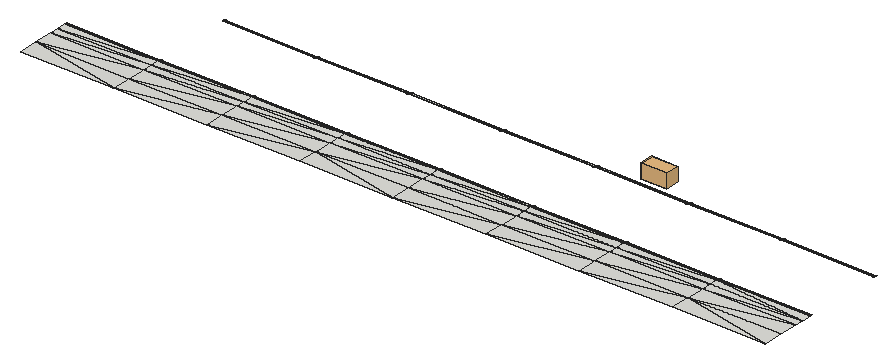
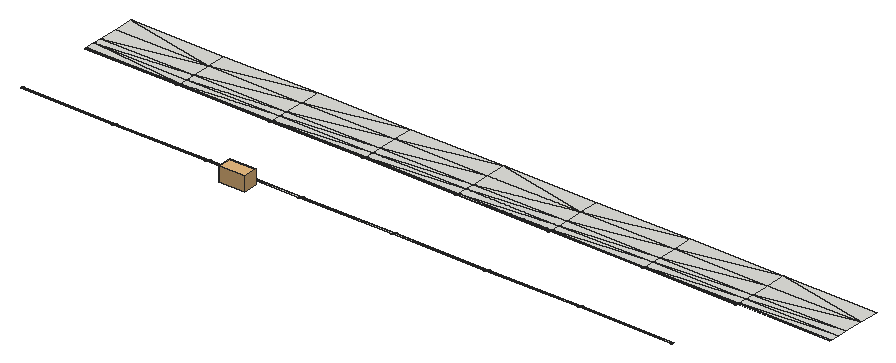
# SketchUp Ruby script. Lengths in inches.
U = 1.inch
M = Sketchup.active_model
def pt(a) = Geom::Point3d.new(a.map { |v| v * U })
def face(e, loops, mat)
  f = e.add_face(loops[0].map { |a| pt(a) })
  loops[1..].each { |l| e.add_face(l.map { |a| pt(a) }).erase! }
  f.material = f.back_material = mat if mat
  f
end
# faces: each face lists its corners as indices into pts; further lists are holes
def faces(e, pts, list, mat = nil) = list.each { |f| face(e, (f[0].is_a?(Array) ? f : [f]).map { |l| l.map { |i| pts[i] } }, mat) }
# xy, xz, yz: faces in a plane at the given z, y or x. An outline is a flat list of corners, or four numbers for a rectangle; further outlines are holes
def ring(l) = l.size == 4 ? [[l[0], l[1]], [l[2], l[1]], [l[2], l[3]], [l[0], l[3]]] : l.each_slice(2).to_a
def flat(e, list, mat, &to3) = list.each { |f| face(e, (f[0].is_a?(Array) ? f : [f]).map { |l| ring(l).map { |u, v| to3.(u, v) } }, mat) }
def xy(e, z, list, mat = nil) = flat(e, list, mat) { |x, y| [x, y, z] }
def xz(e, y, list, mat = nil) = flat(e, list, mat) { |x, z| [x, y, z] }
def yz(e, x, list, mat = nil) = flat(e, list, mat) { |y, z| [x, y, z] }
def lines(e, pts, list) = list.each { |a, b| e.add_line(pt(pts[a]), pt(pts[b])) }
# prism: a flat outline (further loops are holes) pulled along v
def prism(e, loops, v, mat = nil)
  f = face(e, loops, mat); d = Geom::Vector3d.new(v.map { |x| x * U })
  f.pushpull(f.normal.samedirection?(d) ? d.length : -d.length)
end
def box(e, o, s, mat = nil) = prism(e, [[o, [o[0] + s[0], o[1], o[2]], [o[0] + s[0], o[1] + s[1], o[2]], [o[0], o[1] + s[1], o[2]]]], [0, 0, s[2]], mat)
def at(x, y, z, deg = 0) = Geom::Transformation.translation(pt([x, y, z])) * Geom::Transformation.rotation(ORIGIN, Z_AXIS, deg.degrees)
def axes(o, x, y, z) = Geom::Transformation.new([*x, 0, *y, 0, *z, 0, *pt(o).to_a, 1])
def part(name) = M.definitions.add(name)
# library, detail: a bought-in or finely detailed component or shape, given as its bounding box
def library(name, o, s) = part(name).tap { |d| box(d.entities, o, s) }
def detail(e, o, s) = box(e.add_group.entities, o, s)
def put(e, d, t, mat = nil) = e.add_instance(d, t).tap { |i| i.material = mat if mat }
def group(e, t, mat = nil) = e.add_group.tap { |g| g.transformation = t; g.material = mat if mat }.entities
root = M.entities
c1 = library("Ruscus aculeatus 004",[-18.74,-17.86,-1.06],[37.01,36.62,28.95])
xy(root,0.2,[[0,116.21,0.61,116.21,0,116.39],[0.61,116.21,0.61,116.39,0,116.39]])
xy(root,0.37,[[1538.23,281.6,1539,281.6,1538.23,281.84],[1539,281.6,1539,281.84,1538.23,281.84],[1538.23,281.84,1539,281.84,1538.23,285.35],[1539,281.84,1539,285.35,1538.23,285.35],[1538.23,285.35,1539,285.35,1538.23,285.61],
  [1539,285.35,1539,285.61,1538.23,285.61]])
xy(root,0.375,[[1538.36,116.21,1539,116.21,1538.36,116.39],[1539,116.21,1539,116.39,1538.36,116.39],[1538.36,116.39,1539,116.39,1538.36,119.84],[1539,116.39,1539,119.84,1538.36,119.84],[1538.36,119.84,1539,119.84,1538.36,120.23],
  [1539,119.84,1539,120.23,1538.36,120.23]])
p = [[192.375,0,0.22],[192.375,40.18,0.22],[0,40.18,0.2],[0,0,0.2],[384.75,40.18,0.24],[384.75,0,0.24],
  [577.125,40.18,0.26],[577.125,0,0.27],[192.375,78.07,0.22],[0,78.07,0.2],[384.75,78.07,0.24],[577.125,78.07,0.26],
  [192.375,96.84,0.22],[0,96.84,0.2],[384.75,96.84,0.24],[577.125,96.84,0.26],[192.375,115.6,0.22],[0,115.6,0.2],
  [384.75,115.6,0.24],[577.125,115.6,0.26],[0,115.83,0.2],[192.375,115.83,0.22],[384.75,115.83,0.24],[577.125,115.83,0.26],
  [1154.25,115.83,0.33],[1154.25,115.97,0.22],[961.88,115.97,0.2],[961.88,115.83,0.31],[1346.63,115.83,0.35],[1346.63,115.97,0.24],
  [1539,115.83,0.375],[1539,115.97,0.27],[961.875,116.08,0.2],[961.875,116.21,0.31],[769.5,116.21,0.29],[1154.25,116.08,0.22],
  [1154.25,116.21,0.33],[1346.625,116.08,0.24],[1346.625,116.21,0.35],[1538.36,116.08,0.27],[1538.36,116.21,0.375],[192.375,116.21,0.22],
  [192.375,116.39,0.22],[0.61,116.39,0.2],[0.61,116.21,0.2],[384.75,116.39,0.24],[384.75,116.21,0.24],[577.125,116.39,0.26],
  [577.125,116.21,0.26],[0.61,119.84,0.19],[384.75,119.84,0.24],[192.375,119.84,0.22],[577.125,119.84,0.26],[192.375,120.23,0.22],
  [384.75,120.23,0.24],[577.125,120.23,0.26],[577.125,120.47,0.21],[769.5,120.23,0.28],[769.5,120.47,0.23],[961.875,120.23,0.31],
  [961.875,120.47,0.26],[577.125,281.36,0.21],[577.125,281.6,0.26],[384.75,281.6,0.24],[769.5,281.36,0.23],[769.5,281.6,0.28],
  [961.875,281.36,0.25],[384.75,281.84,0.24],[192.375,281.84,0.21],[192.375,281.6,0.21],[577.125,281.84,0.26],[384.75,285.35,0.24],
  [192.375,285.35,0.21],[577.125,285.35,0.26],[192.375,285.61,0.21],[384.75,285.61,0.24],[577.125,285.61,0.26],[1346.625,285.61,0.35],
  [1346.625,285.75,0.24],[1154.25,285.75,0.22],[1154.25,285.61,0.33],[1538.23,285.61,0.37],[1538.23,285.75,0.26],[769.5,0,0.29],
  [769.5,40.18,0.29],[961.875,40.18,0.31],[961.88,0,0.3125],[1154.25,40.18,0.33],[1154.25,0,0.33],[1346.63,40.18,0.35],
  [1346.63,0,0.36],[769.5,78.07,0.29],[961.875,78.07,0.31],[1154.25,78.07,0.33],[1346.63,78.07,0.35],[769.5,96.84,0.29],
  [961.875,96.84,0.31],[1154.25,96.84,0.33],[1346.63,96.84,0.35],[769.5,115.6,0.29],[961.88,115.6,0.31],[1154.25,115.6,0.33],
  [1346.63,115.6,0.35],[769.5,115.83,0.29],[1539,116.08,0.27],[1539,116.21,0.375],[769.5,116.39,0.29],[961.875,116.39,0.31],
  [1154.25,116.39,0.33],[1346.625,116.39,0.35],[769.5,119.84,0.28],[961.875,119.84,0.31],[1154.25,119.84,0.33],[1346.625,119.84,0.35],
  [1154.25,120.23,0.33],[1346.625,120.23,0.35],[1154.25,120.47,0.28],[1346.625,120.47,0.3],[1538.36,120.23,0.375],[1538.36,120.47,0.32],
  [1539,120.23,0.375],[1539,120.47,0.32],[961.875,281.6,0.3],[1154.25,281.36,0.28],[1154.25,281.6,0.33],[1346.63,281.36,0.3],
  [1346.63,281.6,0.35],[1538.23,281.36,0.32],[1538.23,281.6,0.37],[1539,281.36,0.32],[1539,281.6,0.37],[769.5,281.84,0.28],
  [961.875,281.84,0.3],[1154.25,281.84,0.33],[1346.63,281.84,0.35],[1538.23,281.84,0.37],[769.5,285.35,0.28],[961.875,285.35,0.3],
  [1154.25,285.35,0.33],[1346.625,285.35,0.35],[1538.23,285.35,0.37],[769.5,285.61,0.28],[961.875,285.61,0.3],[1539,285.61,0.37],
  [1539,285.75,0.26],[1539,0,0.38],[1539,40.18,0.38],[1539,78.07,0.375],[1539,96.84,0.375],[1539,115.6,0.375],
  [1538.36,116.39,0.375],[1538.36,119.84,0.375]]
faces(root,p,[[0,1,2],[2,3,0],[4,1,0],[0,5,4],[6,4,5],[5,7,6],[8,9,2],[2,1,8],
  [10,8,1],[1,4,10],[11,10,4],[4,6,11],[12,13,9],[9,8,12],[14,12,8],[8,10,14],
  [15,14,10],[10,11,15],[16,17,13],[13,12,16],[18,16,12],[12,14,18],[19,18,14],[14,15,19],
  [20,17,16],[16,21,20],[21,16,18],[18,22,21],[22,18,19],[19,23,22],[24,25,26],[26,27,24],
  [28,29,25],[25,24,28],[30,31,29],[29,28,30],[32,33,34],[33,32,35],[35,36,33],[36,35,37],
  [37,38,36],[37,39,40],[40,38,37],[41,42,43],[43,44,41],[45,42,41],[41,46,45],[47,45,46],
  [46,48,47],[49,43,42],[50,51,42],[42,45,50],[52,50,45],[45,47,52],[53,51,50],[50,54,53],
  [54,50,52],[52,55,54],[56,55,57],[57,58,56],[58,57,59],[59,60,58],[61,62,63],[62,61,64],
  [64,65,62],[65,64,66],[67,68,69],[69,63,67],[70,67,63],[63,62,70],[71,72,68],[68,67,71],
  [73,71,67],[67,70,73],[74,72,71],[71,75,74],[75,71,73],[73,76,75],[77,78,79],[79,80,77],
  [78,77,81],[81,82,78],[83,84,6],[6,7,83],[85,84,83],[83,86,85],[87,85,86],[86,88,87],
  [89,87,88],[88,90,89],[91,11,6],[6,84,91],[92,91,84],[84,85,92],[93,92,85],[85,87,93],
  [94,93,87],[87,89,94],[95,15,11],[11,91,95],[96,95,91],[91,92,96],[97,96,92],[92,93,97],
  [98,97,93],[93,94,98],[99,19,15],[15,95,99],[100,99,95],[95,96,100],[101,100,96],[96,97,101],
  [102,101,97],[97,98,102],[103,23,19],[19,99,103],[103,99,100],[100,27,103],[27,100,101],[101,24,27],
  [24,101,102],[102,28,24],[40,39,104],[104,105,40],[34,106,47],[47,48,34],[107,106,34],[34,33,107],
  [108,107,33],[33,36,108],[109,108,36],[36,38,109],[110,52,47],[47,106,110],[111,110,106],[106,107,111],
  [112,111,107],[107,108,112],[113,112,108],[108,109,113],[57,55,52],[52,110,57],[57,110,111],[111,59,57],
  [59,111,112],[112,114,59],[114,112,113],[113,115,114],[60,59,114],[114,116,60],[116,114,115],[115,117,116],
  [117,115,118],[118,119,117],[119,118,120],[120,121,119],[66,122,65],[122,66,123],[123,124,122],[124,123,125],
  [125,126,124],[125,127,128],[128,126,125],[128,127,129],[129,130,128],[65,131,70],[70,62,65],[132,131,65],
  [65,122,132],[133,132,122],[122,124,133],[134,133,124],[124,126,134],[128,135,134],[134,126,128],[136,73,70],
  [70,131,136],[137,136,131],[131,132,137],[138,137,132],[132,133,138],[139,138,133],[133,134,139],[139,134,135],
  [135,140,139],[141,76,73],[73,136,141],[141,136,137],[137,142,141],[142,137,138],[138,80,142],[80,138,139],
  [139,77,80],[77,139,140],[140,81,77],[82,81,143],[143,144,82],[145,146,89],[89,90,145],[147,94,89],
  [89,146,147],[148,98,94],[94,147,148],[148,149,102],[102,98,148],[149,30,28],[28,102,149],[40,150,109],
  [109,38,40],[113,109,150],[150,151,113],[115,113,151],[151,118,115]])
put(root,c1,axes([1070.49,312.18,1.49],[1.44677,0,0],[0,0.777,0],[0,0,1]))
